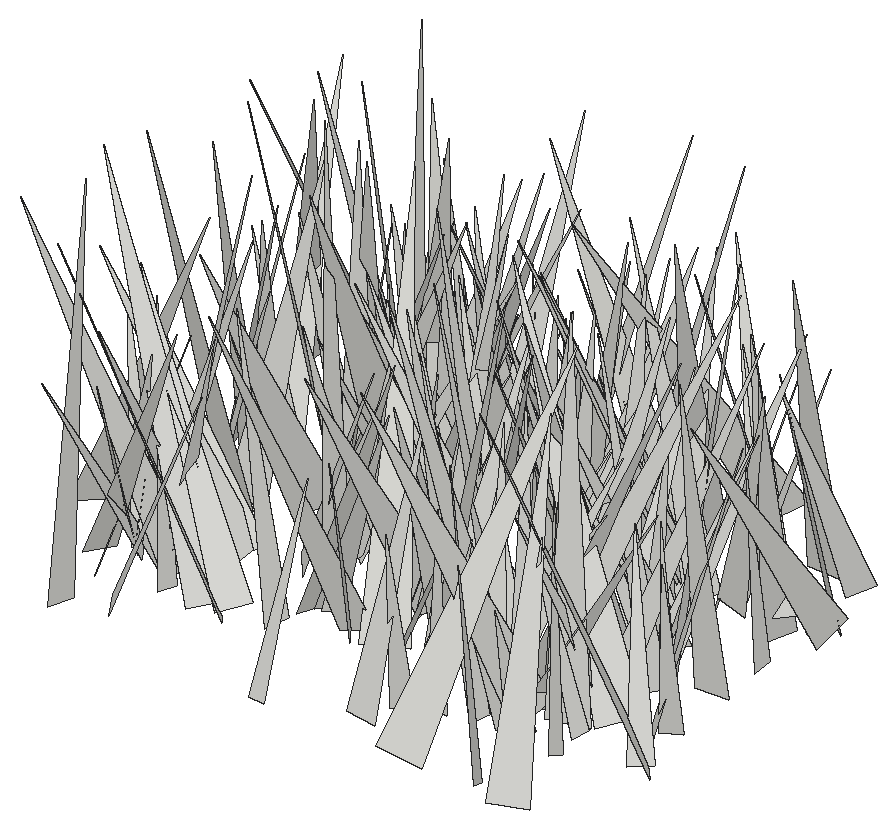
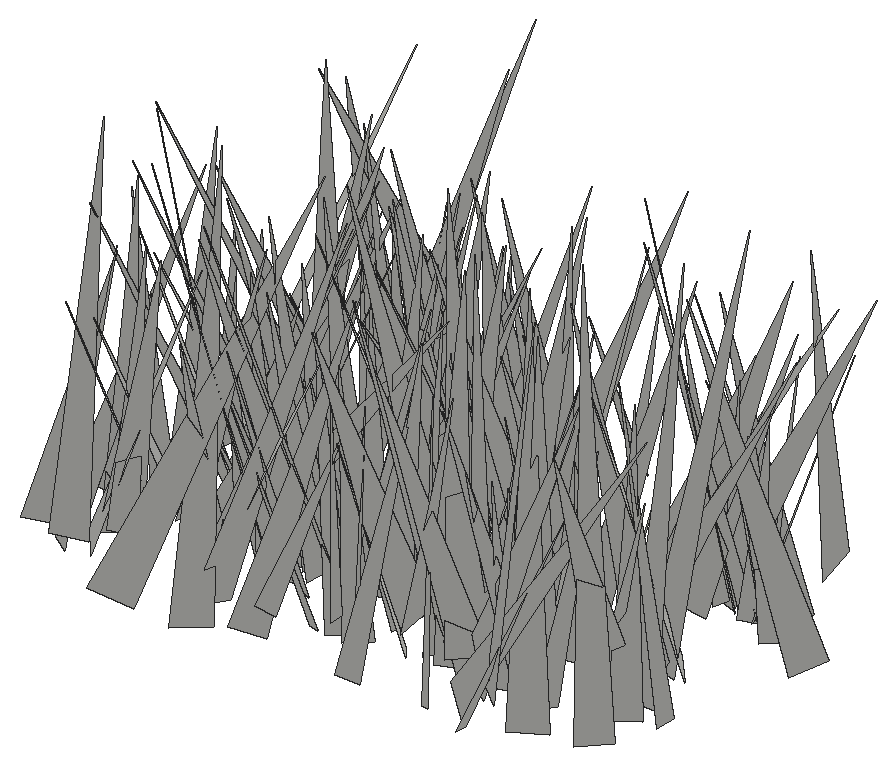
# SketchUp Ruby script. Lengths in inches.
U = 1.inch
M = Sketchup.active_model
def pt(a) = Geom::Point3d.new(a.map { |v| v * U })
def face(e, loops, mat)
  f = e.add_face(loops[0].map { |a| pt(a) })
  loops[1..].each { |l| e.add_face(l.map { |a| pt(a) }).erase! }
  f.material = f.back_material = mat if mat
  f
end
# faces: each face lists its corners as indices into pts; further lists are holes
def faces(e, pts, list, mat = nil) = list.each { |f| face(e, (f[0].is_a?(Array) ? f : [f]).map { |l| l.map { |i| pts[i] } }, mat) }
# xy, xz, yz: faces in a plane at the given z, y or x. An outline is a flat list of corners, or four numbers for a rectangle; further outlines are holes
def ring(l) = l.size == 4 ? [[l[0], l[1]], [l[2], l[1]], [l[2], l[3]], [l[0], l[3]]] : l.each_slice(2).to_a
def flat(e, list, mat, &to3) = list.each { |f| face(e, (f[0].is_a?(Array) ? f : [f]).map { |l| ring(l).map { |u, v| to3.(u, v) } }, mat) }
def xy(e, z, list, mat = nil) = flat(e, list, mat) { |x, y| [x, y, z] }
def xz(e, y, list, mat = nil) = flat(e, list, mat) { |x, z| [x, y, z] }
def yz(e, x, list, mat = nil) = flat(e, list, mat) { |y, z| [x, y, z] }
def lines(e, pts, list) = list.each { |a, b| e.add_line(pt(pts[a]), pt(pts[b])) }
# prism: a flat outline (further loops are holes) pulled along v
def prism(e, loops, v, mat = nil)
  f = face(e, loops, mat); d = Geom::Vector3d.new(v.map { |x| x * U })
  f.pushpull(f.normal.samedirection?(d) ? d.length : -d.length)
end
def box(e, o, s, mat = nil) = prism(e, [[o, [o[0] + s[0], o[1], o[2]], [o[0] + s[0], o[1] + s[1], o[2]], [o[0], o[1] + s[1], o[2]]]], [0, 0, s[2]], mat)
def at(x, y, z, deg = 0) = Geom::Transformation.translation(pt([x, y, z])) * Geom::Transformation.rotation(ORIGIN, Z_AXIS, deg.degrees)
def axes(o, x, y, z) = Geom::Transformation.new([*x, 0, *y, 0, *z, 0, *pt(o).to_a, 1])
def part(name) = M.definitions.add(name)
# library, detail: a bought-in or finely detailed component or shape, given as its bounding box
def library(name, o, s) = part(name).tap { |d| box(d.entities, o, s) }
def detail(e, o, s) = box(e.add_group.entities, o, s)
def put(e, d, t, mat = nil) = e.add_instance(d, t).tap { |i| i.material = mat if mat }
def group(e, t, mat = nil) = e.add_group.tap { |g| g.transformation = t; g.material = mat if mat }.entities
root = M.entities
c1 = part("fur_instance\#9")
p = [[0.8125,0,1.79],[0.67,-0.02,1.48],[0,-0.11,0],[0,0.11,0]]
faces(c1.entities,p,[[0,1,2,3]])
put(root,c1,axes([134.18,167.84,-28.22],[-2.78795,6.31949,0.96814],[6.36227,2.84625,-0.25738],[0.62828,-0.78026,6.90234]))
put(root,c1,axes([122.99,168.23,-28.22],[1.03899,3.82207,0.22987],[3.79032,-1.06041,0.49963],[-0.54276,-0.08876,3.92914]))
put(root,c1,axes([133.25,169.33,-28.22],[2.89571,-2.97183,2.13904],[-3.49598,-3.05481,0.48854],[-1.08874,1.90494,4.12046]))
put(root,c1,axes([132.45,168.38,-28.22],[-5.03149,-1.83162,1.20846],[-2.18082,4.50919,-2.24552],[0.24343,2.5384,4.86091]))
put(root,c1,axes([130.99,173.24,-28.22],[-7.73279,0.49202,2.83462],[1.75633,7.24586,3.53356],[2.27869,-3.91518,6.89581]))
put(root,c1,axes([127.17,170.89,-28.22],[2.03457,-2.99845,1.01926],[-3.06758,-2.16697,-0.25148],[-0.78708,0.69471,3.61482]))
put(root,c1,axes([115.11,170.24,-28.22],[4.3525,2.53578,0.43229],[2.57081,-4.2585,-0.90411],[0.08934,-0.99816,4.9555]))
put(root,c1,axes([126.51,169.47,-28.22],[0.44242,5.64748,1.29703],[5.78226,-0.34572,-0.46699],[0.37666,-1.32609,5.6455]))
put(root,c1,axes([129.2,168.17,-28.22],[-1.94232,7.80928,1.11049],[7.41359,2.19794,-2.48968],[2.69386,-0.41817,7.65238]))
put(root,c1,axes([136.28,172.82,-28.22],[-5.605,-5.08718,0.25266],[-5.09303,5.60246,-0.18084],[0.06544,0.30374,7.56721]))
put(root,c1,axes([113.64,169.36,-28.22],[-7.13651,-0.0123,2.39844],[-0.61978,7.28244,-1.80677],[2.31701,1.91008,6.90402]))
put(root,c1,axes([128.2,171.4375,-28.22],[0.16475,-3.83195,1.51207],[-4.1166,-0.0965,0.20397],[0.15418,1.51796,3.83006]))
put(root,c1,axes([128.04,171.34,-28.22],[2.59266,-2.6088,0.97622],[-2.78019,-2.50569,0.68761],[-0.17141,1.18171,3.61316]))
put(root,c1,axes([131.16,172.06,-28.22],[-0.93338,-7.69941,2.7531],[-7.87622,0.10215,-2.38461],[-2.19672,2.90522,7.38009]))
put(root,c1,axes([113.43,174.09,-28.22],[-3.93384,-2.91751,0.42121],[-2.51987,3.69278,2.04402],[1.52955,-1.41982,4.45073]))
put(root,c1,axes([118.62,171.84,-28.22],[-5.49378,-4.48735,0.1731],[-4.21573,5.05933,-2.64174],[-1.54724,2.14821,6.58325]))
put(root,c1,axes([122.68,174.13,-28.22],[0.32689,-6.93131,1.01824],[-6.72809,-0.59471,-1.88835],[-1.95261,0.88881,6.67713]))
put(root,c1,axes([113.01,174.06,-28.22],[-2.16154,-4.08693,0.6496],[-3.73051,2.24163,1.68984],[1.79115,-0.26331,4.30345]))
put(root,c1,axes([112.38,173.06,-28.22],[5.28357,-2.5058,0.04843],[-2.504,-5.27298,0.35108],[0.10676,0.33794,5.83712]))
put(root,c1,axes([122.54,173.88,-28.22],[-2.98653,-2.99705,1.42564],[-2.58075,3.30304,1.53746],[2.08674,-0.20437,3.94181]))
put(root,c1,axes([129.74,171.98,-28.22],[-6.43885,-0.2283,0.73687],[-0.34147,6.39798,-1.00159],[0.69173,1.03328,6.36457]))
put(root,c1,axes([115.56,173.51,-28.22],[-2.36054,6.29762,2.85628],[6.53149,1.03928,3.10644],[-2.27111,-3.55673,5.96508]))
put(root,c1,axes([115.52,174.82,-28.22],[0.77993,-5.26102,0.56712],[-5.12867,-0.89269,-1.22806],[-1.30258,0.36472,5.1748]))
put(root,c1,axes([113.21,171.87,-28.22],[4.04394,2.43918,0.42992],[2.39305,-4.06014,0.52577],[-0.63852,0.23141,4.69325]))
put(root,c1,axes([133.27,171.58,-28.22],[-4.31752,-0.25034,0.73123],[-0.52227,4.00392,-1.71296],[0.56974,1.77322,3.97108]))
put(root,c1,axes([133.04,173.17,-28.22],[-3.91396,0.19988,0.40503],[0.19284,3.93443,-0.07818],[0.40843,0.05784,3.91828]))
put(root,c1,axes([115.04,173.6,-28.22],[4.73571,-1.08461,0.9225],[-1.0987,-4.82145,-0.02851],[-0.90568,0.17765,4.85824]))
put(root,c1,axes([120.24,172.78,-28.22],[-5.56537,0.35389,1.01892],[0.25962,5.63719,-0.53984],[1.04691,0.48332,5.55042]))
put(root,c1,axes([127.84,171.32,-28.22],[6.62272,2.03005,2.53711],[1.31072,-6.93962,2.13125],[-2.97322,1.46257,6.59085]))
put(root,c1,axes([132.6875,175.29,-28.22],[-4.32918,-1.79601,0.73607],[-1.48596,4.22424,1.56749],[1.24875,-1.19977,4.41706]))
put(root,c1,axes([115.86,172.35,-28.22],[-5.02502,0.15502,0.9974],[-0.08895,4.97687,-1.22169],[1.00545,1.21508,4.87671]))
put(root,c1,axes([129.8125,172.46,-28.22],[-0.91047,5.0165,1.03079],[5.11456,0.83694,0.44447],[-0.2628,-1.09133,5.07905]))
put(root,c1,axes([118.45,172.69,-28.22],[-3.94655,4.7323,0.06828],[4.56087,3.77904,1.70056],[-1.26405,-1.13963,5.92267]))
put(root,c1,axes([120.58,174.375,-28.22],[6.16535,-1.94029,0.16764],[-1.94054,-6.16752,-0.01601],[-0.16472,0.03505,6.46343]))
put(root,c1,axes([135.98,172.77,-28.22],[-2.51117,3.39602,0.58609],[3.43959,2.51478,0.1658],[0.21361,-0.57041,4.22035]))
put(root,c1,axes([117.65,172.45,-28.22],[-4.22364,6.9226,0.63988],[6.72709,3.88063,2.42031],[-1.75445,-1.78585,7.73974]))
put(root,c1,axes([123.51,177.14,-28.22],[6.11084,-2.63091,1.80363],[-1.49433,-5.80472,-3.40432],[-2.81811,-2.62692,5.71618]))
put(root,c1,axes([112.01,174.81,-28.22],[2.04033,-4.0488,0.48109],[-4.03745,-1.93127,0.8697],[0.56854,0.81522,4.44965]))
put(root,c1,axes([132.21,173.53,-28.22],[1.64686,-6.77743,3.62945],[-7.62252,-1.92308,-0.13234],[-1.0018,3.49096,6.97339]))
put(root,c1,axes([120.96,174.77,-28.22],[4.36325,-2.68491,0.18726],[-2.69098,-4.34538,0.39756],[0.04948,0.43666,5.1077]))
put(root,c1,axes([113.86,173.85,-28.22],[3.4737,5.90005,1.74495],[6.11319,-3.08303,-1.74525],[0.69596,-2.36778,6.62052]))
put(root,c1,axes([130.67,173.58,-28.22],[4.72114,-1.50275,0.05764],[-1.46013,-4.53503,1.361],[0.36002,1.31378,4.76394]))
put(root,c1,axes([114.84,173.42,-28.22],[5.7382,5.20942,1.87337],[5.41352,-5.84467,-0.3291],[-1.15821,-1.50876,7.74318]))
put(root,c1,axes([135.37,175.18,-28.22],[1.81522,-3.21568,0.8696],[-3.29805,-1.87418,-0.04607],[-0.46866,0.73395,3.69235]))
put(root,c1,axes([113.28,173.77,-28.22],[-2.88957,-1.62735,2.00469],[-2.2228,3.09866,-0.68855],[1.31385,1.66334,3.24403]))
put(root,c1,axes([129.8,175.67,-28.22],[4.34491,0.59069,1.09524],[0.90101,-4.23706,-1.28924],[-0.85828,-1.45776,4.19106]))
put(root,c1,axes([113.5,174.13,-28.22],[-2.18486,3.79279,1.02862],[3.92891,2.13324,0.47945],[0.08359,-1.13179,4.35074]))
put(root,c1,axes([124.57,176.5,-28.22],[2.86729,-4.50295,0.62999],[-4.43501,-2.93396,-0.78577],[-1.00209,0.10064,5.2802]))
put(root,c1,axes([125.81,176.05,-28.22],[1.75802,-6.33898,1.96931],[-6.51413,-2.03906,-0.74828],[-1.27556,1.67662,6.53555]))
put(root,c1,axes([116.5,175.95,-28.22],[-6.1435,0.43905,0.01492],[0.43419,6.03663,1.1429],[-0.06685,-1.14104,6.05221]))
put(root,c1,axes([127.22,172.36,-28.22],[-5.11664,3.91829,0.85035],[3.38571,4.96082,-2.48663],[2.14782,1.51438,5.94556]))
put(root,c1,axes([129.375,173.9375,-28.22],[-6.96753,-1.64469,0.65915],[-1.76863,6.61713,-2.18437],[0.10697,2.27915,6.81763]))
put(root,c1,axes([129.1,175.46,-28.22],[4.14484,0.5886,1.74948],[0.68446,-4.48393,-0.11303],[-1.71425,-0.36717,4.1849]))
put(root,c1,axes([109.95,175.4375,-28.22],[6.2285,-2.9564,0.62521],[-3.02175,-6.08711,1.31964],[0.01382,1.46019,6.76705]))
put(root,c1,axes([132.35,176.38,-28.22],[-3.35511,-5.27651,0.83113],[-5.27558,3.11951,-1.49198],[-0.83701,1.48869,6.07225]))
put(root,c1,axes([125.19,177.55,-28.22],[7.4678,0.08394,0.57516],[0.2355,-7.21321,-2.00499],[-0.53141,-2.01703,7.1941]))
put(root,c1,axes([133.52,174.7,-28.22],[-7.18183,4.15456,0.03319],[4.14203,7.15453,0.70461],[-0.3242,-0.62648,8.26695]))
put(root,c1,axes([127.3,176.125,-28.22],[2.92691,3.10527,0.26779],[2.82947,-2.4932,-2.01476],[1.3071,-1.55642,3.76168]))
put(root,c1,axes([134.93,175.66,-28.22],[3.01506,-0.72225,2.0256],[-1.00024,-3.559,0.21985],[-1.90373,0.72607,3.09256]))
put(root,c1,axes([116.43,176.07,-28.22],[-4.43376,3.47486,0.22998],[3.34427,4.14468,1.85019],[-0.97128,-1.59146,5.32068]))
put(root,c1,axes([128.35,175.14,-28.22],[0.2906,4.64928,0.9365],[4.41539,0.07727,-1.75374],[1.73123,-0.9775,4.31562]))
put(root,c1,axes([118.38,176.47,-28.22],[3.8282,2.91024,0.83789],[3.01788,-3.55309,-1.44728],[0.25298,-1.65308,4.58585]))
put(root,c1,axes([121.1875,174.66,-28.22],[4.39596,-0.31282,2.17467],[-1.10489,-4.51925,1.5834],[-1.89902,1.90528,4.11281]))
put(root,c1,axes([129.77,174.51,-28.22],[6.72656,-0.08852,1.07497],[-0.40385,-6.50233,1.99163],[-1.00015,2.03024,6.42556]))
put(root,c1,axes([124.09,173.83,-28.22],[-3.14428,7.71271,0.49149],[7.72648,3.12546,0.38342],[-0.17032,-0.59964,8.32018]))
put(root,c1,axes([124.81,173.67,-28.22],[4.98815,3.01806,0.37753],[2.59556,-4.60182,2.49383],[-1.58564,1.9615,5.26983]))
put(root,c1,axes([113.92,178.59,-28.22],[-2.39726,-7.68863,1.50052],[-7.81274,2.46126,0.12966],[0.5725,1.39306,8.05265]))
put(root,c1,axes([129.74,179,-28.22],[0.49777,-7.47829,0.86543],[-7.52286,-0.52678,-0.22508],[-0.28353,0.84808,7.49146]))
put(root,c1,axes([128.32,175.99,-28.22],[-4.17339,1.81444,1.20525],[1.74242,4.34394,-0.50613],[1.30721,0.0026,4.52253]))
put(root,c1,axes([127.62,175.79,-28.22],[-7.81157,-0.92448,1.21309],[-1.13809,7.74743,-1.42443],[1.01538,1.5715,7.73604]))
put(root,c1,axes([119.57,178.18,-28.22],[-4.50462,1.14541,2.32905],[1.86637,4.67145,1.31236],[1.80364,-1.97324,4.45884]))
put(root,c1,axes([135.13,174.32,-28.22],[3.56764,3.88458,0.34534],[3.52617,-3.41301,1.96335],[-1.66594,1.09483,4.89523]))
put(root,c1,axes([126.24,178.28,-28.22],[-6.85321,0.30824,0.48855],[0.41589,6.6696,1.62593],[0.40091,-1.64973,6.66467]))
put(root,c1,axes([116.43,180.02,-28.22],[4.75153,-4.99406,0.9078],[-4.47168,-4.70683,-2.48828],[-2.40183,-1.11663,6.42854]))
put(root,c1,axes([127.79,175.82,-28.22],[-6.2227,2.39174,0.32304],[2.36421,6.22042,-0.51348],[0.48507,0.36431,6.64671]))
put(root,c1,axes([129.9,175.08,-28.22],[3.14457,7.68443,0.45621],[7.56933,-2.99688,-1.69436],[1.40136,-1.05601,8.12822]))
put(root,c1,axes([120.35,175.89,-28.22],[-8.04005,-0.21045,2.18635],[-0.63833,8.16213,-1.56173],[2.10165,1.67397,7.88972]))
put(root,c1,axes([134.71,178.19,-28.22],[0.27233,-6.25887,1.87066],[-6.53155,-0.29195,-0.02597],[-0.1084,1.8677,6.26474]))
put(root,c1,axes([124.5625,178.26,-28.22],[-6.22259,1.31552,1.1088],[1.51746,6.15727,1.21077],[0.81078,-1.42761,6.24382]))
put(root,c1,axes([131.24,177.19,-28.22],[-6.43064,-2.17008,0.24743],[-2.17262,6.27662,-1.4168],[-0.22404,1.42068,6.6374]))
put(root,c1,axes([125.84,174.84,-28.22],[-7.73799,2.57835,1.8542],[1.9672,7.72518,-2.53263],[2.4932,1.90688,7.75308]))
put(root,c1,axes([123.87,178.8,-28.22],[1.97582,-3.11414,0.08334],[-3.10691,-1.9626,0.3224],[0.22782,0.24287,3.67393]))
put(root,c1,axes([125.46,179.28,-28.22],[-4.70083,-1.74871,0.0814],[-1.70109,4.61801,0.97093],[0.41342,-0.88228,4.92068]))
put(root,c1,axes([123.92,176.7,-28.22],[6.62959,-1.41825,2.66639],[-1.99694,-6.88369,1.30369],[-2.26567,1.91728,6.65307]))
put(root,c1,axes([131.54,178.86,-28.22],[-3.46593,0.7925,0.89611],[1.04093,3.35143,1.06213],[0.58952,-1.25841,3.39303]))
put(root,c1,axes([121.25,178.5625,-28.22],[4.26328,-1.39926,0.74192],[-1.39292,-4.32659,-0.15583],[-0.75375,0.08115,4.48433]))
put(root,c1,axes([128.49,178.46,-28.22],[2.27684,-3.73592,1.683],[-3.94498,-2.51908,-0.25488],[-1.10756,1.29258,4.36763]))
put(root,c1,axes([132.07,176.08,-28.22],[2.81698,6.47491,0.35167],[6.46114,-2.77024,-0.75032],[0.54938,-0.62035,7.02117]))
put(root,c1,axes([118.45,178.87,-28.22],[-6.42891,-4.93695,1.78859],[-5.18873,6.40682,-0.96596],[0.80598,1.86616,8.04806]))
put(root,c1,axes([115.14,179.98,-28.22],[-3.15969,-2.10838,0.70871],[-1.88389,3.19122,1.09464],[1.18257,-0.54957,3.6374]))
put(root,c1,axes([126.1875,179.35,-28.22],[4.31409,-4.88001,1.43702],[-5.06352,-4.30068,0.59646],[-0.49016,1.47666,6.48614]))
put(root,c1,axes([126.44,178.29,-28.22],[0.74077,3.76285,1.03817],[3.63302,-0.27816,-1.5841],[1.42759,-1.24465,3.49262]))
put(root,c1,axes([133.8125,177.04,-28.22],[5.36611,5.59511,2.05394],[5.5109,-5.71038,1.15783],[-2.27022,-0.63666,7.66549]))
put(root,c1,axes([132.17,178.31,-28.22],[4.29759,3.17988,0.45483],[3.21134,-4.23507,-0.73441],[0.07624,-0.86047,5.29543]))
put(root,c1,axes([131.875,179.9,-28.22],[0.21984,-5.04241,1.33274],[-4.72838,-0.75562,-2.0789],[-2.20101,1.11963,4.59917]))
put(root,c1,axes([129.07,177.74,-28.22],[0.34617,6.42334,1.62872],[6.51894,-0.03728,-1.2385],[1.18972,-1.66468,6.31231]))
put(root,c1,axes([122.25,179.36,-28.22],[-3.35147,5.54659,2.9979],[6.27053,3.28643,0.92965],[0.65767,-3.06906,6.41348]))
put(root,c1,axes([112.78,180.92,-28.22],[-1.7083,-7.51191,1.45388],[-7.48357,1.95063,1.28533],[1.59333,1.10775,7.59572]))
put(root,c1,axes([122.73,177.05,-28.22],[4.46685,2.95329,0.59597],[2.75098,-4.43263,1.34675],[-1.2285,0.81223,5.18275]))
put(root,c1,axes([133.11,177.11,-28.22],[0.1109,6.16383,0.84068],[5.38265,-0.51661,3.07768],[-3.11876,-0.67243,5.34163]))
put(root,c1,axes([118.08,178.7,-28.22],[6.24865,-3.61776,1.18124],[-3.80474,-5.99015,1.78079],[-0.08657,2.13519,6.99733]))
put(root,c1,axes([119.06,178.51,-28.22],[4.17015,5.48726,0.52169],[5.30168,-3.81404,-2.26221],[1.50809,-1.76505,6.51019]))
put(root,c1,axes([114.14,178.74,-28.22],[-0.87926,6.56228,2.62812],[6.83144,1.46959,-1.38397],[1.81713,-2.34956,6.47466]))
put(root,c1,axes([118.73,181.67,-28.22],[-4.18199,-2.55213,0.91155],[-1.98836,4.02848,2.15666],[1.84139,-1.44616,4.39901]))
put(root,c1,axes([117.49,183.11,-28.22],[5.60712,-6.07402,0.33398],[-5.83929,-5.5015,-2.02021],[-1.70529,-1.13347,8.01575]))
put(root,c1,axes([120.39,179.32,-28.22],[2.58495,3.56171,0.23056],[3.43761,-2.40789,-1.34382],[0.96012,-0.96809,4.1907]))
put(root,c1,axes([130.77,179.82,-28.22],[0.06663,3.86387,1.64805],[4.18879,0.06273,-0.31643],[0.31563,-1.6482,3.85147]))
put(root,c1,axes([122.97,182.04,-27.1],[4.57924,-4.33247,0.58798],[-4.22206,-4.60304,-1.03525],[-1.13589,-0.35667,6.21836]))
put(root,c1,axes([122.39,180.85,-28.22],[5.22033,-0.21574,2.13038],[0.1303,-5.5713,-0.88347],[-2.13731,-0.86658,5.14955]))
put(root,c1,axes([113.28,178.08,-28.22],[4.49985,4.45709,1.03745],[4.28289,-4.6143,1.2473],[-1.61209,0.1822,6.20956]))
put(root,c1,axes([127.2,179.82,-28.22],[-4.36102,2.95909,2.58691],[3.11538,4.95832,-0.41976],[2.39639,-1.06094,5.25343]))
put(root,c1,axes([135.36,183.9,-28.22],[5.96418,-2.86813,1.57613],[-1.66285,-5.47776,-3.67572],[-2.81874,-2.83722,5.50334]))
put(root,c1,axes([132.4,178.12,-28.22],[1.99959,6.47326,0.24716],[6.43471,-1.95494,-0.85747],[0.74746,-0.48749,6.72058]))
put(root,c1,axes([134.93,180.63,-28.22],[3.59976,0.06174,1.80471],[0.19659,-4.01441,-0.2548],[-1.79504,-0.31584,3.59126]))
put(root,c1,axes([111.39,181.39,-28.22],[5.83398,1.13984,1.03884],[1.35175,-5.73614,-1.2974],[-0.74243,-1.48703,5.80098]))
put(root,c1,axes([129.89,182.72,-27.1],[-6.83596,-2.73328,0.53057],[-2.58478,6.75268,1.48423],[1.035,-1.18879,7.21098]))
put(root,c1,axes([132.79,181.65,-27.1],[0.54307,-5.39112,1.14857],[-5.29865,-0.1925,1.60174],[1.51911,1.25582,5.17624]))
put(root,c1,axes([130.34,180.12,-28.22],[-5.00631,-5.98003,0.73957],[-5.22244,3.82659,-4.41068],[-3.00563,3.31169,6.43193]))
put(root,c1,axes([129.98,182.63,-27.1],[-5.72076,-3.26575,0.35826],[-3.1922,5.6955,0.94426],[0.77675,-0.64548,6.51924]))
put(root,c1,axes([119.83,181.62,-28.22],[8.10386,-2.02713,0.06413],[-2.02706,-8.10412,-0.01624],[-0.06615,-0.00019,8.35354]))
put(root,c1,axes([125.62,180.41,-28.22],[3.88682,0.49651,1.01606],[0.42112,-4.01087,0.34905],[-1.04955,0.22945,3.90283]))
put(root,c1,axes([112.5625,182.14,-28.22],[3.52243,-4.25283,0.7835],[-4.27225,-3.57882,-0.21878],[-0.66956,0.46198,5.5178]))
put(root,c1,axes([130.27,178.91,-28.22],[-0.5351,4.97369,0.08314],[4.96853,0.53845,-0.2337],[0.24128,-0.05757,4.99693]))
put(root,c1,axes([134.07,182.59,-28.22],[5.38586,-3.00561,1.16634],[-2.8404,-5.49795,-1.05176],[-1.52519,-0.37466,6.07741]))
put(root,c1,axes([125.49,180.41,-28.22],[-0.24087,4.17753,0.95098],[3.88217,0.61574,-1.72155],[1.81241,-0.76371,3.81393]))
put(root,c1,axes([118.09,182.4,-27.1],[2.18541,-3.04998,0.78828],[-3.02604,-2.29919,-0.50659],[-0.87571,0.3334,3.71777]))
put(root,c1,axes([116.02,182.24,-28.22],[6.51578,-0.90085,0.09034],[-0.89347,-6.50413,-0.41604],[-0.1463,-0.39981,6.56459]))
put(root,c1,axes([130.17,182.36,-28.22],[-4.34148,-1.68145,0.56308],[-1.64517,4.37512,0.38015],[0.66161,-0.1544,4.64018]))
put(root,c1,axes([116.8,180.6875,-28.22],[4.32331,2.64676,1.47041],[2.57631,-4.56233,0.63737],[-1.59061,-0.19566,5.02892]))
put(root,c1,axes([118.98,183.24,-27.1],[1.51991,-3.61395,0.26794],[-3.4425,-1.53065,-1.11749],[-1.13207,-0.1975,3.75792]))
put(root,c1,axes([113.92,181.42,-27.1],[-3.79892,0.58903,0.61511],[0.5899,3.84804,-0.04166],[0.61427,-0.05255,3.84409]))
put(root,c1,axes([126.1,181.69,-27.1],[6.14943,-1.42717,1.61929],[-1.52874,-6.3314,0.22535],[-1.52376,0.59247,6.30885]))
put(root,c1,axes([118.09,183.49,-27.1],[6.18232,-5.30847,0.7026],[-5.32058,-6.21081,-0.10875],[-0.60412,0.37485,8.14795]))
put(root,c1,axes([119.89,181.4,-27.1],[5.9079,4.20697,0.32991],[4.15488,-5.69984,-1.72033],[0.73785,-1.5887,7.04573]))
put(root,c1,axes([120.04,181.42,-27.1],[-3.12705,-1.8127,0.50032],[-1.87769,2.95706,-1.02213],[-0.10232,1.13341,3.46693]))
put(root,c1,axes([116.66,181.59,-27.1],[-5.0872,2.66073,2.45988],[2.85923,5.55214,-0.09239],[2.22604,-1.05084,5.74025]))
put(root,c1,axes([124.34,182.31,-28.22],[-6.25427,-0.78477,1.30734],[-0.71032,6.38344,0.43371],[1.34924,-0.27711,6.28838]))
put(root,c1,axes([123.83,183.5,-28.22],[0.90872,-5.0896,0.45336],[-4.90772,-0.74115,1.51668],[1.42262,0.69427,4.94262]))
put(root,c1,axes([117.77,181.41,-28.22],[-2.49672,2.92464,0.96124],[2.97957,2.60694,-0.1927],[0.77439,-0.6012,3.84057]))
put(root,c1,axes([119.48,182.88,-28.22],[1.5026,-5.2869,1.47769],[-5.48951,-1.44343,0.41772],[0.01326,1.53554,5.48039]))
put(root,c1,axes([122.9,181.6,-27.1],[-2.01026,5.06538,1.49078],[5.275,1.85579,0.80751],[-0.23431,-1.67916,5.38954]))
put(root,c1,axes([127.86,181.87,-28.22],[-1.18817,5.57554,2.26119],[5.96275,1.39894,-0.31626],[0.80332,-2.13721,5.69196]))
put(root,c1,axes([131.7,181.57,-27.1],[-6.69944,1.03913,0.45559],[1.00559,6.70154,-0.49804],[0.5255,0.42362,6.76123]))
put(root,c1,axes([115.23,183.11,-28.22],[-4.62696,1.13691,1.70574],[1.48296,4.76376,0.84751],[1.41525,-1.27471,4.68861]))
put(root,c1,axes([120.16,182.1875,-28.22],[5.58768,-4.04107,3.86555],[-4.58295,-6.44048,-0.10822],[-3.20457,2.16447,6.89498]))
put(root,c1,axes([114.61,184.8,-28.22],[1.80193,-7.44469,0.50754],[-7.36471,-1.69029,1.35351],[1.20089,0.80465,7.53912]))
put(root,c1,axes([125.62,182.21,-27.1],[5.24089,-0.83273,1.62957],[-1.05437,-5.41429,0.62423],[-1.49573,0.89885,5.2698]))
put(root,c1,axes([118.52,180.95,-28.22],[-4.46885,1.59045,1.08144],[1.18804,4.43404,-1.61169],[1.51249,1.21632,4.46123]))
put(root,c1,axes([126.2,181.99,-27.1],[0.11042,6.13884,2.00494],[6.14565,0.51615,-1.91884],[1.98398,-1.94051,5.83229]))
put(root,c1,axes([132.14,181.03,-28.22],[4.1336,3.03674,0.5342],[2.87698,-4.11997,1.15876],[-1.10914,0.6308,4.99657]))
put(root,c1,axes([111.09,185.61,-27.1],[8.00988,-2.00577,0.3429],[-1.833,-7.71682,-2.32157],[-0.88363,-2.17404,7.92412]))
put(root,c1,axes([119.03,181.74,-27.1],[2.99088,7.34321,2.70362],[7.47912,-3.53374,1.32409],[-2.30112,-1.94104,7.81761]))
put(root,c1,axes([122.98,183.5,-28.22],[3.01124,-3.84874,1.35887],[-4.04465,-3.04041,0.35153],[-0.54781,1.29229,4.87409]))
put(root,c1,axes([135.09,184.46,-28.22],[-3.17607,-4.40082,1.193],[-4.40846,3.33508,0.56622],[1.16445,0.62283,5.3976]))
put(root,c1,axes([126.3125,185.3,-28.22],[2.95346,-5.37759,1.21149],[-5.08452,-3.18852,-1.75785],[-2.12927,0.1548,5.87804]))
put(root,c1,axes([134.58,182.26,-27.1],[-1.36293,4.52681,0.55653],[4.38086,1.13777,1.47406],[-1.26877,-0.93423,4.49185]))
put(root,c1,axes([117.8,182.05,-27.1],[-4.10668,0.43412,1.0008],[0.12519,4.05996,-1.24738],[1.0837,1.17608,3.93666]))
put(root,c1,axes([132.625,184.14,-27.1],[1.7038,-4.78318,1.39426],[-4.94528,-1.80274,-0.14134],[-0.60574,1.26373,5.0756]))
put(root,c1,axes([128.01,186.2,-28.22],[7.64117,-3.1953,0.94942],[-2.87226,-7.51641,-2.18001],[-1.69158,-1.67105,7.9903]))
put(root,c1,axes([119.65,182.93,-27.1],[3.29943,5.39851,1.49465],[5.593,-3.07886,-1.22601],[0.31023,-1.9081,6.20701]))
put(root,c1,axes([133.89,185.49,-27.1],[0.64901,-7.30772,0.94418],[-7.33385,-0.54888,0.79295],[0.71332,1.00569,7.2935]))
put(root,c1,axes([121.28,183.06,-28.22],[3.16954,2.48643,0.53995],[2.54162,-3.13416,-0.48689],[-0.1185,-0.71733,3.99891]))
put(root,c1,axes([132.78,182.24,-27.1],[3.07177,3.42083,0.35758],[3.42072,-3.08846,0.16062],[-0.35863,-0.15826,4.59478]))
put(root,c1,axes([135.51,185.26,-27.1],[3.42862,-3.42654,1.21049],[-3.04602,-3.61734,-1.61199],[-1.98197,-0.36822,4.57144]))
put(root,c1,axes([127.79,182.44,-27.1],[5.42391,5.6075,1.42758],[5.74422,-5.4537,-0.40246],[-0.69711,-1.3092,7.79108]))
put(root,c1,axes([115.7,183.51,-27.1],[1.80806,-4.3936,1.6396],[-4.55829,-1.23367,1.72079],[1.10181,2.10605,4.4285]))
put(root,c1,axes([134.39,183.69,-28.22],[-5.08452,-4.09315,0.88657],[-4.17476,4.84247,-1.58557],[-0.33349,1.78573,6.33184]))
put(root,c1,axes([126.9,181.79,-28.22],[1.99951,5.4557,0.6063],[5.41529,-2.06607,0.73224],[-0.89823,-0.31139,5.76424]))
put(root,c1,axes([128.56,184.54,-28.22],[-8.04315,1.60644,1.39343],[1.83623,7.99603,1.38066],[1.07265,-1.64234,8.08496]))
put(root,c1,axes([123.3,184.28,-27.1],[3.69206,0.52175,1.19179],[0.74035,-3.79133,-0.63373],[-1.0698,-0.8231,3.6745]))
put(root,c1,axes([118.42,185.6,-28.22],[-2.8265,-4.26887,1.57231],[-3.66111,3.23328,2.19698],[2.70032,-0.08465,4.62446]))
put(root,c1,axes([128.84,183.79,-27.1],[-4.50374,-2.5863,0.2222],[-2.55985,4.35118,-1.23954],[-0.43072,1.18335,5.04343]))
put(root,c1,axes([121.65,185.73,-28.22],[-0.22883,-5.12281,0.23524],[-5.12454,0.23734,0.18366],[0.19416,0.22665,5.12463]))
put(root,c1,axes([130.17,187.9,-27.1],[4.91107,-6.51993,1.1851],[-5.42781,-4.80392,-3.93621],[-3.80168,-1.5638,7.15082]))
put(root,c1,axes([124.76,183.64,-28.22],[2.48404,3.35431,0.63876],[3.34518,-2.23213,-1.28736],[0.685,-1.26336,3.97047]))
put(root,c1,axes([121.08,182.94,-27.1],[-5.72971,0.10944,0.75393],[-0.02545,5.68949,-1.01935],[0.7614,1.01378,5.63937]))
put(root,c1,axes([118.26,183.31,-28.22],[-3.06653,-6.21678,2.70439],[-6.51984,1.89062,-3.04678],[-1.85842,3.62531,6.22648]))
put(root,c1,axes([118.04,183.1,-28.22],[-3.15581,4.82371,2.67558],[4.59437,4.00448,-1.80054],[3.05265,-1.04019,5.47589]))
put(root,c1,axes([130.61,181.55,-28.22],[0.42359,6.38348,0.10104],[6.1795,-0.43539,1.60081],[-1.60398,0.00839,6.194]))
put(root,c1,axes([124.99,182.22,-27.1],[4.48947,6.23838,0.89691],[6.27438,-4.52789,0.08708],[-0.59503,-0.67674,7.68539]))
put(root,c1,axes([115.95,185.17,-27.1],[-4.21383,-5.23135,2.06774],[-5.35043,4.52497,0.54449],[1.7365,1.24763,6.69529]))
put(root,c1,axes([122.43,181.15,-28.22],[-6.29891,4.40553,1.36932],[3.82289,6.28157,-2.62437],[2.58248,1.44677,7.22479]))
put(root,c1,axes([133.375,183.1875,-27.1],[-3.60307,5.2202,0.86904],[5.28801,3.51043,0.83765],[-0.20649,-1.18922,6.28736]))
put(root,c1,axes([125.52,185.33,-27.1],[0.6602,-3.48398,0.63366],[-3.31771,-0.83389,-1.12823],[-1.23791,0.37685,3.36171]))
put(root,c1,axes([113.64,181.39,-27.1],[-5.02723,4.35262,0.08247],[4.19421,4.87628,-1.68986],[1.1665,1.22544,6.43138]))
put(root,c1,axes([116.55,185.99,-28.22],[-4.29176,-1.39668,0.34406],[-1.22552,4.11722,1.42648],[0.75311,-1.25938,4.28195]))
put(root,c1,axes([122.49,184.21,-27.1],[2.78644,2.89477,1.9564],[3.12581,-3.18339,0.25829],[-1.56092,-1.20736,4.00964]))
put(root,c1,axes([117.87,184.58,-28.22],[-4.67528,-5.85921,0.505],[-5.43274,4.05599,-3.23694],[-2.25181,2.37953,6.76097]))
